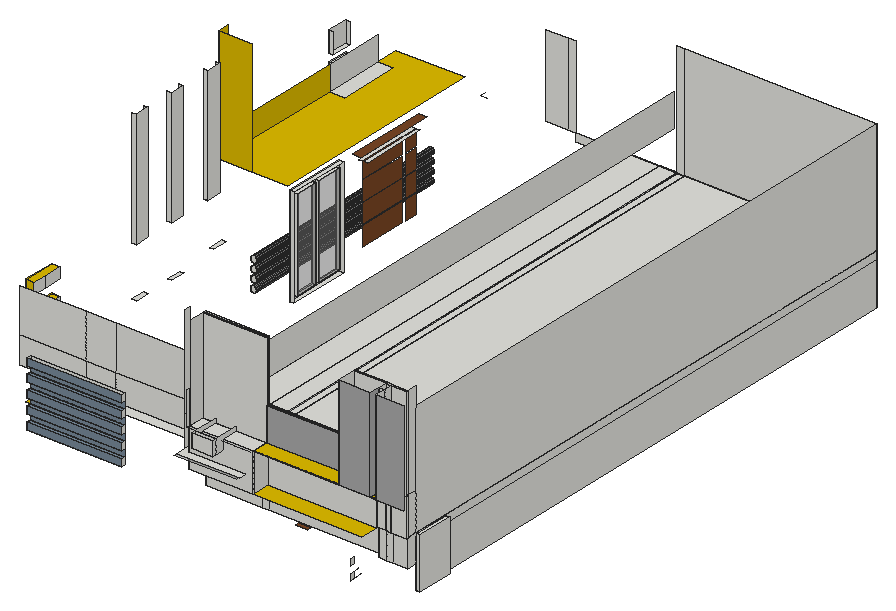
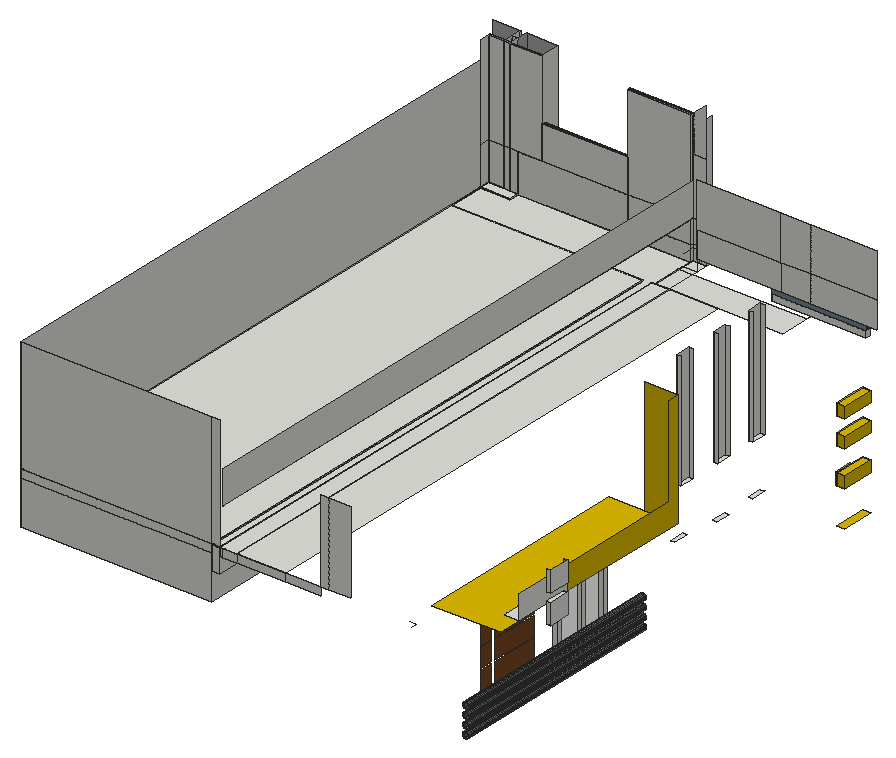
# SketchUp Ruby script. Lengths in inches.
U = 1.inch
M = Sketchup.active_model
def pt(a) = Geom::Point3d.new(a.map { |v| v * U })
def face(e, loops, mat)
  f = e.add_face(loops[0].map { |a| pt(a) })
  loops[1..].each { |l| e.add_face(l.map { |a| pt(a) }).erase! }
  f.material = f.back_material = mat if mat
  f
end
# faces: each face lists its corners as indices into pts; further lists are holes
def faces(e, pts, list, mat = nil) = list.each { |f| face(e, (f[0].is_a?(Array) ? f : [f]).map { |l| l.map { |i| pts[i] } }, mat) }
# xy, xz, yz: faces in a plane at the given z, y or x. An outline is a flat list of corners, or four numbers for a rectangle; further outlines are holes
def ring(l) = l.size == 4 ? [[l[0], l[1]], [l[2], l[1]], [l[2], l[3]], [l[0], l[3]]] : l.each_slice(2).to_a
def flat(e, list, mat, &to3) = list.each { |f| face(e, (f[0].is_a?(Array) ? f : [f]).map { |l| ring(l).map { |u, v| to3.(u, v) } }, mat) }
def xy(e, z, list, mat = nil) = flat(e, list, mat) { |x, y| [x, y, z] }
def xz(e, y, list, mat = nil) = flat(e, list, mat) { |x, z| [x, y, z] }
def yz(e, x, list, mat = nil) = flat(e, list, mat) { |y, z| [x, y, z] }
def lines(e, pts, list) = list.each { |a, b| e.add_line(pt(pts[a]), pt(pts[b])) }
# prism: a flat outline (further loops are holes) pulled along v
def prism(e, loops, v, mat = nil)
  f = face(e, loops, mat); d = Geom::Vector3d.new(v.map { |x| x * U })
  f.pushpull(f.normal.samedirection?(d) ? d.length : -d.length)
end
def box(e, o, s, mat = nil) = prism(e, [[o, [o[0] + s[0], o[1], o[2]], [o[0] + s[0], o[1] + s[1], o[2]], [o[0], o[1] + s[1], o[2]]]], [0, 0, s[2]], mat)
def at(x, y, z, deg = 0) = Geom::Transformation.translation(pt([x, y, z])) * Geom::Transformation.rotation(ORIGIN, Z_AXIS, deg.degrees)
def axes(o, x, y, z) = Geom::Transformation.new([*x, 0, *y, 0, *z, 0, *pt(o).to_a, 1])
def part(name) = M.definitions.add(name)
# library, detail: a bought-in or finely detailed component or shape, given as its bounding box
def library(name, o, s) = part(name).tap { |d| box(d.entities, o, s) }
def detail(e, o, s) = box(e.add_group.entities, o, s)
def put(e, d, t, mat = nil) = e.add_instance(d, t).tap { |i| i.material = mat if mat }
def group(e, t, mat = nil) = e.add_group.tap { |g| g.transformation = t; g.material = mat if mat }.entities
root = M.entities
M.materials.add("[0046_Gold]").color = [221, 186, 0]
M.materials.add("[0110_LightSlateGray]").color = [119, 136, 153]
M.materials.add("[0132_LightGray]").color = [169, 169, 169]
M.materials.add("[0133_Gray]").color = [128, 128, 128]
M.materials.add("[Translucent Glass Gray]").color = [128, 128, 128]
M.materials["[Translucent Glass Gray]"].alpha = 0.5
M.materials.add("[Wood Veneer 01]").color = [120, 70, 37]
xy(root,175.8125,[[128.78,328.14,131.78,373.08]])
xy(root,178.8125,[[128.78,331.14,131.78,348.35],[128.78,351.04,131.78,370.08]])
xy(root,179.37,[[88,138.31,94,162.08]],"[0046_Gold]")
xy(root,199.84,[[320.34,93.62,329.34,96.62]],"[Wood Veneer 01]")
xy(root,205.375,[[427.31,70.06,427.68,96.62],[427.68,70.06,430.18,96.62]])
xy(root,205.625,[[94,148.68,94.81,162.08]])
xy(root,205.625,[[88,138.31,94,162.08]],"[0046_Gold]")
xy(root,213.9,[[94,148.68,94.81,162.08]])
xy(root,213.9,[[88,138.31,94,162.08]],"[0046_Gold]")
xy(root,218.9,[[106,245.52,109,256.27]])
xy(root,219.9,[[106,212.89,109,223.64]])
xy(root,220.21,[[312.51,89.5,360.51,96.62]],"[Wood Veneer 01]")
xy(root,222.46,[[106,283.77,109,294.52]])
xy(root,222.49,[[405.67,62.68,427.31,70.06]])
xy(root,225.3125,[[279.43,62.68,279.43,95.5,282.09,95.5,282.09,489.31,287.5,489.31,287.5,96.62,427.31,96.62,427.31,70.06,405.67,70.06,405.67,62.68]])
xy(root,226.21,[[306.51,89.5,366.51,95.5]])
xy(root,227.92,[[162.79,46.06,231.72,49.06]],"[0110_LightSlateGray]")
xy(root,231.46,[[88,138.31,94,162.08]],"[0046_Gold]")
xy(root,232.84,[[162.79,46.06,231.72,49.06]],"[0110_LightSlateGray]")
xy(root,238.22,[[125.78,394.87,128.78,442.87],[128.78,394.87,131.78,442.87]])
xy(root,238.36,[[162.79,46.06,231.72,49.06]],"[0110_LightSlateGray]")
xy(root,239.74,[[88,138.31,94,162.08]],"[0046_Gold]")
xy(root,242.5,[[279.43,47.62,279.43,49.06,279.47,49.06,279.47,60.93,279.43,60.93,279.43,61.06,326.02,61.06,326.02,47.62],[279.43,61.06,321.29,62.68],[321.29,61.06,326.02,62.68],[326.02,61.06,405.67,62.68],[279.43,62.68,405.67,62.68,405.67,70.06,427.31,70.06,427.31,96.62,287.5,96.62,287.5,489.31,282.09,489.31,282.09,95.5,279.43,95.5],
  [405.67,62.68,427.31,70.06],[427.31,70.06,430.18,96.62]])
xy(root,242.5,[[326.02,47.37,405.67,61.06]],"[0046_Gold]")
xy(root,242.875,[[233.78,95.5,269.16,489.31],[269.16,95.5,282.09,489.31],[287.5,96.62,427.31,489.31]])
xy(root,243,[[279.43,49.06,279.47,60.93],[269.16,60.93,279.43,61.06],[269.16,61.06,279.43,70.06],[405.67,61.06,411.96,62.68],[411.96,61.06,416.22,62.68],
  [416.22,61.06,427.31,62.68],[405.67,62.68,427.31,70.06],[269.16,70.06,279.43,73.87],[186.6,73.87,269.16,95.5],[269.16,73.87,279.43,95.5]])
xy(root,243.28,[[162.79,46.06,231.72,49.06]],"[0110_LightSlateGray]")
xy(root,244.22,[[125.78,388.87,131.78,448.87]],"[Wood Veneer 01]")
xy(root,245.52,[[128.78,331.14,131.78,348.35],[128.78,351.04,131.78,370.08]])
xy(root,248.52,[[128.78,328.14,131.78,373.08]])
xy(root,248.8,[[162.79,46.06,231.72,49.06]],"[0110_LightSlateGray]")
xy(root,249.21,[[70.87,436.12,73.87,451.12]])
xy(root,250.96,[[88,138.31,94,162.08]],"[0046_Gold]")
xy(root,253.71,[[162.79,46.06,231.72,49.06]],"[0110_LightSlateGray]")
xy(root,253.9,[[275.6,41.62,321.29,61.06],[279.43,61.06,321.29,62.68]])
xy(root,253.9,[[275.6,38.62,321.29,41.62]],"[Translucent Glass Gray]")
xy(root,255.04,[[82,422.6,93.12,466.21]])
xy(root,255.04,[[82,322.08,82,422.6,93.12,422.6,93.12,466.21,82,466.21,82,483.47,131.78,483.47,131.78,322.08]],"[0046_Gold]")
xy(root,256.71,[[106,212.89,109,223.64],[106,244.77,109,255.52],[106,278.27,109,289.02]])
xy(root,259.23,[[162.79,46.06,231.72,49.06]],"[0110_LightSlateGray]")
xy(root,259.24,[[88,138.31,94,162.08]],"[0046_Gold]")
xy(root,263.14,[[288.75,38.62,303.875,41.62],[288.75,41.62,303.875,61.06],[288.75,61.06,303.875,62.68]])
xy(root,264.15,[[162.79,46.06,231.72,49.06]],"[0110_LightSlateGray]")
xy(root,264.21,[[70.87,436.12,73.87,451.12]])
xy(root,269.67,[[162.79,46.06,231.72,49.06]],"[0110_LightSlateGray]")
xy(root,270.27,[[70.87,436.12,73.87,451.12]])
xy(root,270.5625,[[388.7,47.37,405.67,48.18],[405.67,47.37,411.96,48.18],[279.43,47.62,279.43,49.06,279.47,49.06,279.47,60.18,326.02,60.18,326.02,47.62],[388.7,48.18,405.67,61.06],[405.67,48.18,411.96,61.06],
  [279.43,49.06,279.47,60.18],[411.96,55.06,416.22,61.06],[279.43,60.18,279.47,61.06],[279.47,60.18,326.02,60.81],[326.02,60.18,388.7,61.06],
  [279.47,60.81,288.75,61.06],[288.75,60.81,303.875,61.06],[303.875,60.81,326.02,61.06],[279.43,61.06,279.47,62.68],[279.47,61.06,288.75,61.18],
  [288.75,61.06,303.875,61.18],[303.875,61.06,326.02,61.18],[326.02,61.06,388.7,62.68],[388.7,61.06,405.67,61.68],[405.67,61.06,411.96,61.68],
  [411.96,61.06,416.22,62.68],[416.22,61.06,427.31,62.68],[279.47,61.18,288.75,61.31],[288.75,61.18,303.875,61.31],[303.875,61.18,326.02,61.31],
  [279.47,61.31,288.75,62.68],[288.75,61.31,303.875,62.68],[303.875,61.31,326.02,62.68],[388.7,61.68,405.67,62.68],[405.67,61.68,411.96,62.68],
  [279.43,62.68,279.47,489.31]])
xy(root,270.5625,[[326.02,47.37,388.7,48.18],[411.96,47.37,416.22,48.18],[326.02,48.18,388.7,60.18],[411.96,48.18,416.22,55.06]],"[0046_Gold]")
xz(root,38.62,[[288.75,263.14,303.875,273.2]])
xz(root,41.62,[[288.75,263.14,303.875,273.2]])
xz(root,46.06,[[162.79,227.92,231.72,232.84],[162.79,238.36,231.72,243.28],[162.79,248.8,231.72,253.71],[162.79,259.23,231.72,264.15],[162.79,269.67,231.72,274.59]],"[0110_LightSlateGray]")
xz(root,47.37,[[388.7,270.5625,411.96,339],[416.22,270.5625,436.31,339]],"[0132_LightGray]")
xz(root,47.62,[[279.43,242.5,326.02,270.5625]])
xz(root,49.06,[[162.79,227.92,231.72,232.84],[162.79,238.36,231.72,243.28],[279.43,242.5,279.47,243],[162.79,248.8,231.72,253.71],[162.79,259.23,231.72,264.15],
  [162.79,269.67,231.72,274.59],[279.43,270.5625,279.47,339]])
xz(root,49.06,[[162.79,232.84,231.72,238.36],[162.79,243.28,231.72,248.8],[162.79,253.71,231.72,259.23],[162.79,264.15,231.72,269.67]],"[0110_LightSlateGray]")
xz(root,55.06,[[411.96,270.5,416.22,270.5625],[411.96,270.5625,416.22,339]])
xz(root,60.18,[[279.47,270.5625,326.02,339]])
xz(root,60.18,[[326.02,270.5625,388.7,294.8125]],"[0132_LightGray]")
xz(root,60.93,[[279.43,242.5,279.47,243]])
xz(root,61.06,[[279.43,242.5,321.29,253.9],[321.29,242.5,326.02,242.5,326.02,270.5625,303.875,270.5625,303.875,263.14,288.75,263.14,288.75,270.5625,279.43,270.5625,279.43,253.9,321.29,253.9],[326.02,242.5,405.67,270.5625],[269.16,243,269.5,251.375],[269.5,243,275.6,251.375],
  [275.6,243,279.43,251.375],[405.67,243,411.96,270.5625],[411.96,243,416.22,270.5625],[416.22,243,427.31,270.5625],[269.16,251.375,269.5,270.5625],
  [269.5,251.375,275.6,251.375,275.6,253.9,279.43,253.9,279.43,270.5625,269.5,270.5625],[275.6,251.375,279.43,253.9],[288.75,263.14,303.875,270.5625],[269.16,270.5625,269.5,312.4375],[269.5,270.5625,279.43,312.4375],
  [326.02,270.5625,388.7,294.8125],[411.96,270.5625,416.22,339],[416.22,270.5625,427.31,339]])
xz(root,61.18,[[279.47,270.5625,326.02,339]])
xz(root,61.31,[[279.47,270.5625,326.02,339]])
xz(root,61.68,[[388.7,270.5625,411.96,339]])
xz(root,62.68,[[405.67,222.49,411.96,242.5],[411.96,222.49,416.22,242.5],[416.22,222.49,427.31,242.5],[279.43,225.3125,321.29,242.5],[321.29,225.3125,326.02,242.5],
  [326.02,225.3125,405.67,242.5],[279.43,242.5,321.29,253.9],[321.29,242.5,321.29,253.9,279.43,253.9,279.43,270.5625,288.75,270.5625,288.75,263.14,303.875,263.14,303.875,270.5625,326.02,270.5625,326.02,242.5],[326.02,242.5,405.67,270.5625],[405.67,242.5,411.96,243],
  [411.96,242.5,416.22,243],[416.22,242.5,427.31,243],[405.67,243,411.96,270.5625],[411.96,243,416.22,270.5625],[416.22,243,427.31,270.5625],
  [288.75,263.14,303.875,270.5625],[279.47,270.5625,326.02,339],[326.02,270.5625,388.7,294.8125],[388.7,270.5625,411.96,339],[411.96,270.5625,416.22,339],
  [416.22,270.5625,427.31,339]])
xz(root,70.06,[[427.31,205.375,430.18,242.5],[405.67,222.49,427.31,225.3125],[405.67,225.3125,427.31,242.5],[405.67,242.5,427.31,242.875],[405.67,242.875,427.31,243],
  [138.64,251.375,186.6,270.5625],[186.6,251.375,208.53,270.5625],[208.53,251.375,269.16,270.5625],[138.64,270.5625,186.6,303],[186.6,270.5625,208.53,303],
  [208.53,270.5625,269.16,303]])
xz(root,95.5,[[279.43,225.3125,282.09,242.5],[279.43,242.5,282.09,242.875],[269.16,242.875,279.43,243]])
xz(root,96.62,[[427.31,205.375,430.18,237.125],[287.5,225.3125,312.51,242.5],[312.51,225.3125,360.51,242.5],[360.51,225.3125,427.31,242.5],[427.31,237.125,430.18,242.5],
  [287.5,242.5,312.51,242.875],[312.51,242.5,360.51,242.875],[360.51,242.5,427.31,242.875]])
xz(root,96.62,[[312.51,205.375,360.51,220.21]],"[Wood Veneer 01]")
xz(root,138.31,[[88,205.625,94,213.9],[88,231.46,94,239.74],[88,250.96,94,259.24]],"[0046_Gold]")
xz(root,148.68,[[94,205.625,94.81,213.9]])
xz(root,162.08,[[94,205.625,94.81,213.9]])
xz(root,162.08,[[88,205.625,94,213.9],[88,231.46,94,239.74],[88,250.96,94,259.24]],"[0046_Gold]")
xz(root,212.89,[[106,256.71,109,341.65]])
xz(root,223.64,[[106,256.71,109,341.65]])
xz(root,244.77,[[106,256.71,109,341.65]])
xz(root,255.52,[[106,256.71,109,341.65]])
xz(root,278.27,[[106,256.71,109,341.65]])
xz(root,289.02,[[106,256.71,109,341.65]])
xz(root,321.79,[[107.24,176.74,107.82,176.82,108.37,177.04,108.83,177.4,109.1875,177.86,109.41,178.41,109.49,178.99,109.41,179.57,109.1875,180.11,108.83,180.58,108.37,180.9375,107.82,181.16,107.24,181.24,106.66,181.16,106.12,180.9375,105.65,180.58,105.29,180.11,105.07,179.57,104.99,178.99,105.07,178.41,105.29,177.86,105.65,177.4,106.12,177.04,106.66,176.82]])
xz(root,322.08,[[107.24,183.24,107.82,183.32,108.37,183.54,108.83,183.9,109.1875,184.36,109.41,184.91,109.49,185.49,109.41,186.07,109.1875,186.61,108.83,187.08,108.37,187.4375,107.82,187.66,107.24,187.74,106.66,187.66,106.12,187.4375,106,187.35,106,183.63,106.12,183.54,106.66,183.32],[106,183.63,106,187.35,105.65,187.08,105.29,186.61,105.07,186.07,104.99,185.49,105.07,184.91,105.29,184.36,105.65,183.9],[107.24,189.74,107.82,189.82,108.37,190.04,108.83,190.4,109.1875,190.86,109.41,191.41,109.49,191.99,109.41,192.57,109.1875,193.11,108.83,193.58,108.37,193.9375,107.82,194.16,107.24,194.24,106.66,194.16,106.12,193.9375,106,193.85,106,190.13,106.12,190.04,106.66,189.82],[106,190.13,106,193.85,105.65,193.58,105.29,193.11,105.07,192.57,104.99,191.99,105.07,191.41,105.29,190.86,105.65,190.4],[107.24,196.24,107.82,196.32,108.37,196.54,108.83,196.9,109.1875,197.36,109.41,197.91,109.49,198.49,109.41,199.07,109.1875,199.61,108.83,200.08,108.37,200.4375,107.82,200.66,107.24,200.74,106.66,200.66,106.12,200.4375,106,200.35,106,196.63,106.12,196.54,106.66,196.32],
  [106,196.63,106,200.35,105.65,200.08,105.29,199.61,105.07,199.07,104.99,198.49,105.07,197.91,105.29,197.36,105.65,196.9]])
xz(root,322.08,[[82,255.04,106,339]],"[0046_Gold]")
xz(root,328.14,[[128.78,175.8125,131.78,248.52]])
xz(root,331.14,[[128.78,178.8125,131.78,245.52]])
xz(root,348.35,[[128.78,178.8125,131.78,245.52]])
xz(root,351.04,[[128.78,178.8125,131.78,245.52]])
xz(root,370.08,[[128.78,178.8125,131.78,245.52]])
xz(root,373.08,[[128.78,175.8125,131.78,248.52]])
xz(root,436.12,[[70.87,249.21,73.87,264.21],[70.87,270.27,73.87,285.27]])
xz(root,451.12,[[70.87,249.21,73.87,264.21],[70.87,270.27,73.87,285.27]])
xz(root,489.31,[[287.5,205.375,427.31,237.125],[282.09,225.3125,287.5,242.5],[208.53,237.125,208.53,243,269.16,243,269.16,242.875,233.78,242.875,233.78,237.125],[233.78,237.125,269.16,242.875],[269.16,237.125,279.43,242.875],
  [279.43,237.125,282.09,242.875],[287.5,237.125,427.31,242.875],[282.09,242.5,287.5,242.875],[269.16,242.875,279.43,243],[279.43,242.875,282.09,243],
  [282.09,242.875,287.5,243],[287.5,242.875,427.31,243],[186.6,243,202.62,303],[202.62,243,208.53,303],[282.09,243,287.5,325.9375],
  [287.5,243,427.31,325.9375]])
yz(root,70.87,[[436.12,249.21,451.12,264.21],[436.12,270.27,451.12,285.27]])
yz(root,82,[[422.6,255.04,466.21,272.6]])
yz(root,82,[[322.08,255.04,322.08,339,329.95,339,329.95,272.6,422.6,272.6,422.6,255.04]],"[0046_Gold]")
yz(root,88,[[138.31,205.625,162.08,213.9],[138.31,231.46,162.08,239.74],[138.31,250.96,162.08,259.24]],"[0046_Gold]")
yz(root,94,[[138.31,205.625,148.68,213.9],[148.68,205.625,162.08,213.9],[138.31,231.46,148.68,239.74],[148.68,231.46,162.08,239.74],[138.31,250.96,148.68,259.24],
  [148.68,250.96,162.08,259.24]])
yz(root,94.81,[[148.68,205.625,162.08,213.9]])
yz(root,109,[[212.89,256.71,223.64,341.65],[244.77,256.71,255.52,341.65],[278.27,256.71,289.02,341.65]])
yz(root,128.78,[[[328.14,175.8125,373.08,248.52],[351.04,178.8125,370.08,245.52],[331.14,178.8125,348.35,245.52]]])
yz(root,128.78,[[394.87,182.1,430.4,195.83],[433.39,182.1,442.87,195.83],[394.87,196.97,430.4,210.71],[433.39,196.97,442.87,210.71],[394.87,211.85,430.4,225.58],
  [433.39,211.85,442.87,225.58],[394.87,226.72,430.4,238.22],[433.39,226.72,442.87,238.22]],"[Wood Veneer 01]")
yz(root,131.78,[[331.14,178.8125,348.35,245.52],[351.04,178.8125,370.08,245.52]],"[Translucent Glass Gray]")
yz(root,162.79,[[46.06,227.92,49.06,232.84],[46.06,238.36,49.06,243.28],[46.06,248.8,49.06,253.71],[46.06,259.23,49.06,264.15],[46.06,269.67,49.06,274.59]])
yz(root,231.72,[[46.06,227.92,49.06,232.84],[46.06,238.36,49.06,243.28],[46.06,248.8,49.06,253.71],[46.06,259.23,49.06,264.15],[46.06,269.67,49.06,274.59]])
yz(root,269.16,[[95.5,242.875,489.31,243],[56.62,243,61.06,270.5625],[61.06,251.375,70.06,270.5625],[56.62,270.5625,61.06,339]])
yz(root,279.43,[[62.68,225.3125,70.06,242.5],[70.06,225.3125,73.87,242.5],[73.87,225.3125,95.5,242.5],[47.62,242.5,47.62,251.375,61.06,251.375,61.06,243,49.06,243,49.06,242.5],[60.93,242.5,61.06,243],
  [61.06,242.5,62.68,243],[62.68,242.5,70.06,243],[70.06,242.5,73.87,242.875],[73.87,242.5,95.5,242.875],[70.06,242.875,73.87,243],
  [73.87,242.875,95.5,243],[61.06,243,62.68,251.375],[47.62,251.375,61.06,270.5625],[61.06,251.375,62.68,253.9],[61.06,253.9,62.68,270.5625],
  [45.87,270.5625,47.62,294.8125],[47.62,270.5625,49.06,294.8125],[49.06,270.5625,60.18,294.8125],[60.18,270.5625,61.06,294.8125],[61.06,270.5625,489.31,294.8125]])
yz(root,279.47,[[49.06,242.5,60.93,243],[49.06,270.5625,60.18,339],[60.18,270.5625,60.81,339],[60.81,270.5625,61.18,339],[61.18,270.5625,61.31,339],
  [61.31,270.5625,62.68,339]])
yz(root,282.09,[[95.5,225.3125,489.31,242.5],[95.5,242.5,489.31,242.875]])
yz(root,287.5,[[96.62,205.375,489.31,225.3125],[96.62,225.3125,489.31,242.5],[96.62,242.5,489.31,242.875]])
yz(root,288.75,[[38.62,263.14,41.62,273.2],[41.62,263.14,61.06,273.2],[61.06,263.14,62.68,270.5625]])
yz(root,303.875,[[38.62,263.14,41.62,273.2],[41.62,263.14,61.06,273.2],[61.06,263.14,62.68,270.5625]])
yz(root,321.29,[[61.06,242.5,62.68,253.9]])
yz(root,326.02,[[47.37,242.5,47.62,270.5625],[47.62,242.5,48.18,270.5625],[48.18,242.5,61.06,270.5625],[61.06,242.5,62.68,270.5625],[60.18,270.5625,60.81,294.8125],
  [60.81,270.5625,61.06,294.8125],[61.06,270.5625,61.18,294.8125],[61.18,270.5625,61.31,294.8125],[61.31,270.5625,62.68,294.8125]])
yz(root,360.51,[[93.62,177.72,96.62,182.38],[93.62,187.33,96.62,191.96]])
yz(root,388.7,[[47.37,270.5625,47.37,339,61.68,339,61.68,294.8125,60.18,294.8125,60.18,270.5625],[60.18,270.5625,61.06,294.8125],[61.06,270.5625,61.68,294.8125],[61.68,270.5625,62.68,294.8125]])
yz(root,405.67,[[62.68,225.3125,70.06,242.5],[61.06,242.5,62.68,243],[62.68,242.5,70.06,243],[61.06,243,62.68,270.5625]])
yz(root,405.67,[[62.68,222.49,70.06,225.3125]],"[0046_Gold]")
yz(root,411.96,[[61.06,243,62.68,270.5625],[55.06,270.5625,61.06,339],[61.06,270.5625,61.68,339],[61.68,270.5625,62.68,339]])
yz(root,411.96,[[47.37,270.5625,55.06,339]],"[0132_LightGray]")
yz(root,416.22,[[61.06,243,62.68,270.5625],[47.37,270.5625,48.18,339],[48.18,270.5625,55.06,339],[55.06,270.5625,61.06,339],[61.06,270.5625,62.68,339]])
yz(root,427.31,[[70.06,205.375,96.62,225.3125],[96.62,205.375,489.31,237.125],[62.68,222.49,70.06,242.5],[70.06,225.3125,96.62,242.5],[96.62,237.125,489.31,242.875],
  [62.68,242.5,70.06,243],[70.06,242.5,96.62,242.875],[70.06,242.875,489.31,243],[61.06,243,62.68,270.5625],[62.68,243,70.06,270.5625],
  [70.06,243,489.31,325.9375],[61.06,270.5625,62.68,339],[62.68,270.5625,70.06,339]])
yz(root,430.18,[[70.06,205.375,96.62,242.5]])
p = [[106.66,483.47,176.82],[107.24,483.47,176.74],[107.24,321.79,176.74],[106.66,321.79,176.82],[107.82,483.47,176.82],[107.82,321.79,176.82],
  [106.12,483.47,177.04],[106.12,321.79,177.04],[108.37,483.47,177.04],[108.37,321.79,177.04],[105.65,483.47,177.4],[105.65,321.79,177.4],
  [108.83,483.47,177.4],[108.83,321.79,177.4],[105.29,483.47,177.86],[105.29,321.79,177.86],[109.1875,483.47,177.86],[109.1875,321.79,177.86],
  [105.07,483.47,178.41],[105.07,321.79,178.41],[109.41,483.47,178.41],[109.41,321.79,178.41],[104.99,483.47,178.99],[104.99,321.79,178.99],
  [109.49,483.47,178.99],[109.49,321.79,178.99],[105.07,483.47,179.57],[105.07,321.79,179.57],[109.41,483.47,179.57],[109.41,321.79,179.57],
  [105.29,483.47,180.11],[105.29,321.79,180.11],[109.1875,483.47,180.11],[109.1875,321.79,180.11],[105.65,483.47,180.58],[105.65,321.79,180.58],
  [108.83,483.47,180.58],[108.83,321.79,180.58],[106.12,483.47,180.9375],[106.12,321.79,180.9375],[108.37,483.47,180.9375],[108.37,321.79,180.9375],
  [106.66,483.47,181.16],[106.66,321.79,181.16],[107.82,483.47,181.16],[107.82,321.79,181.16],[107.24,483.47,181.24],[107.24,321.79,181.24],
  [106.66,483.47,183.32],[107.24,483.47,183.24],[107.24,322.08,183.24],[106.66,322.08,183.32],[107.82,483.47,183.32],[107.82,322.08,183.32],
  [106.12,483.47,183.54],[106.12,322.08,183.54],[108.37,483.47,183.54],[108.37,322.08,183.54],[105.65,483.47,183.9],[106,322.08,183.63],
  [105.65,322.08,183.9],[108.83,483.47,183.9],[108.83,322.08,183.9],[105.29,483.47,184.36],[105.29,322.08,184.36],[109.1875,483.47,184.36],
  [109.1875,322.08,184.36],[105.07,483.47,184.91],[105.07,322.08,184.91],[109.41,483.47,184.91],[109.41,322.08,184.91],[104.99,483.47,185.49],
  [104.99,322.08,185.49],[109.49,483.47,185.49],[109.49,322.08,185.49],[105.07,483.47,186.07],[105.07,322.08,186.07],[109.41,483.47,186.07],
  [109.41,322.08,186.07],[105.29,483.47,186.61],[105.29,322.08,186.61],[109.1875,483.47,186.61],[109.1875,322.08,186.61],[105.65,483.47,187.08],
  [105.65,322.08,187.08],[108.83,483.47,187.08],[108.83,322.08,187.08],[106.12,483.47,187.4375],[106,322.08,187.35],[106.12,322.08,187.4375],
  [108.37,483.47,187.4375],[108.37,322.08,187.4375],[106.66,483.47,187.66],[106.66,322.08,187.66],[107.82,483.47,187.66],[107.82,322.08,187.66],
  [107.24,483.47,187.74],[107.24,322.08,187.74],[106.66,483.47,189.82],[107.24,483.47,189.74],[107.24,322.08,189.74],[106.66,322.08,189.82],
  [107.82,483.47,189.82],[107.82,322.08,189.82],[106.12,483.47,190.04],[106.12,322.08,190.04],[108.37,483.47,190.04],[108.37,322.08,190.04],
  [105.65,483.47,190.4],[106,322.08,190.13],[105.65,322.08,190.4],[108.83,483.47,190.4],[108.83,322.08,190.4],[105.29,483.47,190.86],
  [105.29,322.08,190.86],[109.1875,483.47,190.86],[109.1875,322.08,190.86],[105.07,483.47,191.41],[105.07,322.08,191.41],[109.41,483.47,191.41],
  [109.41,322.08,191.41],[104.99,483.47,191.99],[104.99,322.08,191.99],[109.49,483.47,191.99],[109.49,322.08,191.99],[105.07,483.47,192.57],
  [105.07,322.08,192.57],[109.41,483.47,192.57],[109.41,322.08,192.57],[105.29,483.47,193.11],[105.29,322.08,193.11],[109.1875,483.47,193.11],
  [109.1875,322.08,193.11],[105.65,483.47,193.58],[105.65,322.08,193.58],[108.83,483.47,193.58],[108.83,322.08,193.58],[106.12,483.47,193.9375],
  [106,322.08,193.85],[106.12,322.08,193.9375],[108.37,483.47,193.9375],[108.37,322.08,193.9375],[106.66,483.47,194.16],[106.66,322.08,194.16],
  [107.82,483.47,194.16],[107.82,322.08,194.16],[107.24,483.47,194.24],[107.24,322.08,194.24],[106.66,483.47,196.32],[107.24,483.47,196.24],
  [107.24,322.08,196.24],[106.66,322.08,196.32],[107.82,483.47,196.32],[107.82,322.08,196.32],[106.12,483.47,196.54],[106.12,322.08,196.54],
  [108.37,483.47,196.54],[108.37,322.08,196.54],[105.65,483.47,196.9],[106,322.08,196.63],[105.65,322.08,196.9],[108.83,483.47,196.9],
  [108.83,322.08,196.9],[105.29,483.47,197.36],[105.29,322.08,197.36],[109.1875,483.47,197.36],[109.1875,322.08,197.36],[105.07,483.47,197.91],
  [105.07,322.08,197.91],[109.41,483.47,197.91],[109.41,322.08,197.91],[104.99,483.47,198.49],[104.99,322.08,198.49],[109.49,483.47,198.49],
  [109.49,322.08,198.49],[105.07,483.47,199.07],[105.07,322.08,199.07],[109.41,483.47,199.07],[109.41,322.08,199.07],[105.29,483.47,199.61],
  [105.29,322.08,199.61],[109.1875,483.47,199.61],[109.1875,322.08,199.61],[105.65,483.47,200.08],[105.65,322.08,200.08],[108.83,483.47,200.08],
  [108.83,322.08,200.08],[106.12,483.47,200.4375],[106,322.08,200.35],[106.12,322.08,200.4375],[108.37,483.47,200.4375],[108.37,322.08,200.4375],
  [106.66,483.47,200.66],[106.66,322.08,200.66],[107.82,483.47,200.66],[107.82,322.08,200.66],[107.24,483.47,200.74],[107.24,322.08,200.74],
  [360.51,96.62,182.38],[364.17,96.62,186.28],[362.21,96.62,179.54],[365.88,96.62,183.4375],[360.51,96.62,177.72],[186.6,70.06,243],
  [186.6,73.87,243],[70.06,60.93,243],[70.06,61.06,243],[138.64,489.31,243],[138.64,494.25,243],[279.43,70.06,251.375],
  [279.43,62.68,251.375],[411.96,55.06,270.5],[411.96,47.62,270.5],[416.22,55.06,270.5],[416.22,47.62,270.5],[279.43,45.87,270.5625],
  [326.02,45.87,270.5625],[269.16,70.06,251.375],[269.16,70.06,243],[143.81,489.31,243]]
faces(root,p,[[0,1,2,3],[1,4,5,2],[6,0,3,7],[4,8,9,5],[10,6,7,11],[8,12,13,9],[14,10,11,15],[12,16,17,13],
  [18,14,15,19],[16,20,21,17],[22,18,19,23],[20,24,25,21],[26,22,23,27],[24,28,29,25],[30,26,27,31],[28,32,33,29],
  [34,30,31,35],[32,36,37,33],[38,34,35,39],[36,40,41,37],[42,38,39,43],[40,44,45,41],[46,42,43,47],[44,46,47,45],
  [48,49,50,51],[49,52,53,50],[54,48,51,55],[52,56,57,53],[58,54,55,59,60],[56,61,62,57],[63,58,60,64],[61,65,66,62],
  [67,63,64,68],[65,69,70,66],[71,67,68,72],[69,73,74,70],[75,71,72,76],[73,77,78,74],[79,75,76,80],[77,81,82,78],
  [83,79,80,84],[81,85,86,82],[87,83,84,88,89],[85,90,91,86],[92,87,89,93],[90,94,95,91],[96,92,93,97],[94,96,97,95],
  [98,99,100,101],[99,102,103,100],[104,98,101,105],[102,106,107,103],[108,104,105,109,110],[106,111,112,107],[113,108,110,114],[111,115,116,112],
  [117,113,114,118],[115,119,120,116],[121,117,118,122],[119,123,124,120],[125,121,122,126],[123,127,128,124],[129,125,126,130],[127,131,132,128],
  [133,129,130,134],[131,135,136,132],[137,133,134,138,139],[135,140,141,136],[142,137,139,143],[140,144,145,141],[146,142,143,147],[144,146,147,145],
  [148,149,150,151],[149,152,153,150],[154,148,151,155],[152,156,157,153],[158,154,155,159,160],[156,161,162,157],[163,158,160,164],[161,165,166,162],
  [167,163,164,168],[165,169,170,166],[171,167,168,172],[169,173,174,170],[175,171,172,176],[173,177,178,174],[179,175,176,180],[177,181,182,178],
  [183,179,180,184],[181,185,186,182],[187,183,184,188,189],[185,190,191,186],[192,187,189,193],[190,194,195,191],[196,192,193,197],[194,196,197,195]],"[0133_Gray]")
lines(root,p,[[198,199],[200,201],[202,200],[203,204],[205,206],[207,208],[209,210],[211,212],[213,214],[215,216],[217,218],[207,219]])
